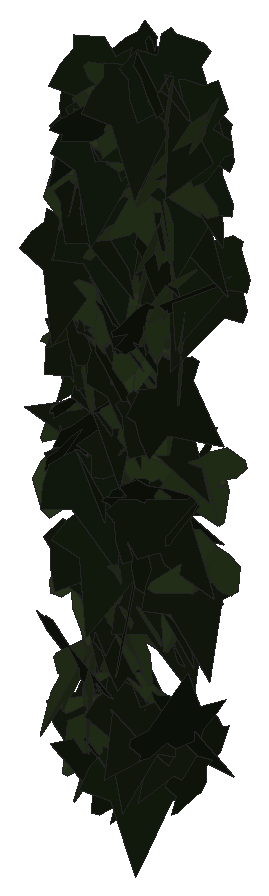
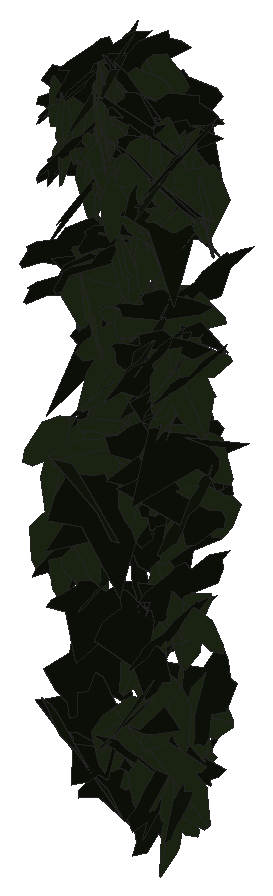
# SketchUp Ruby script. Lengths in inches.
U = 1.inch
M = Sketchup.active_model
def pt(a) = Geom::Point3d.new(a.map { |v| v * U })
def face(e, loops, mat)
  f = e.add_face(loops[0].map { |a| pt(a) })
  loops[1..].each { |l| e.add_face(l.map { |a| pt(a) }).erase! }
  f.material = f.back_material = mat if mat
  f
end
# faces: each face lists its corners as indices into pts; further lists are holes
def faces(e, pts, list, mat = nil) = list.each { |f| face(e, (f[0].is_a?(Array) ? f : [f]).map { |l| l.map { |i| pts[i] } }, mat) }
# xy, xz, yz: faces in a plane at the given z, y or x. An outline is a flat list of corners, or four numbers for a rectangle; further outlines are holes
def ring(l) = l.size == 4 ? [[l[0], l[1]], [l[2], l[1]], [l[2], l[3]], [l[0], l[3]]] : l.each_slice(2).to_a
def flat(e, list, mat, &to3) = list.each { |f| face(e, (f[0].is_a?(Array) ? f : [f]).map { |l| ring(l).map { |u, v| to3.(u, v) } }, mat) }
def xy(e, z, list, mat = nil) = flat(e, list, mat) { |x, y| [x, y, z] }
def xz(e, y, list, mat = nil) = flat(e, list, mat) { |x, z| [x, y, z] }
def yz(e, x, list, mat = nil) = flat(e, list, mat) { |y, z| [x, y, z] }
def lines(e, pts, list) = list.each { |a, b| e.add_line(pt(pts[a]), pt(pts[b])) }
# prism: a flat outline (further loops are holes) pulled along v
def prism(e, loops, v, mat = nil)
  f = face(e, loops, mat); d = Geom::Vector3d.new(v.map { |x| x * U })
  f.pushpull(f.normal.samedirection?(d) ? d.length : -d.length)
end
def box(e, o, s, mat = nil) = prism(e, [[o, [o[0] + s[0], o[1], o[2]], [o[0] + s[0], o[1] + s[1], o[2]], [o[0], o[1] + s[1], o[2]]]], [0, 0, s[2]], mat)
def at(x, y, z, deg = 0) = Geom::Transformation.translation(pt([x, y, z])) * Geom::Transformation.rotation(ORIGIN, Z_AXIS, deg.degrees)
def axes(o, x, y, z) = Geom::Transformation.new([*x, 0, *y, 0, *z, 0, *pt(o).to_a, 1])
def part(name) = M.definitions.add(name)
# library, detail: a bought-in or finely detailed component or shape, given as its bounding box
def library(name, o, s) = part(name).tap { |d| box(d.entities, o, s) }
def detail(e, o, s) = box(e.add_group.entities, o, s)
def put(e, d, t, mat = nil) = e.add_instance(d, t).tap { |i| i.material = mat if mat }
def group(e, t, mat = nil) = e.add_group.tap { |g| g.transformation = t; g.material = mat if mat }.entities
root = M.entities
M.materials.add("efeu1").color = [18, 25, 13]
M.materials.add("efeu2").color = [43, 57, 29]
c1 = part("ivyleaf_10")
p = [[0,0.5,-0.03],[-0.0625,2.02,-0.43],[-0.19,2.01,-0.46],[-0.54,1.05,-0.29],[-0.52,0.625,-0.18],[-0.83,0.76,-0.28],
  [-1.16,0.64,-0.33],[-1.15,0.33,-0.24],[-0.77,-0.39,0.02],[-0.3,-0.51,0.16],[0.04,-0.48,0.23],[-0.02,2.01,-0.4375],
  [-0.06,2.01,-0.43],[0.04,-0.49,0.23],[0.67,-0.49,0.14],[1.38,0.36,-0.2],[1.375,0.51,-0.24],[0.81,0.65,-0.19],
  [0.62,0.59,-0.15],[0.6,1.09,-0.28],[0.5,1.23,-0.31]]
faces(c1.entities,p,[[0,1,2,3,4,5,6,7,8,9,10],[11,12,0,13,14,15,16,17,18,19,20]],"efeu2")
c2 = part("ivyleaf_9")
p = [[1.54,2.16,1.25],[1.36,2.04,1.19],[-0.21,0.99,0.68],[-0.71,1.11,0.82],[-0.85,0.86,0.67],[-0.8,0.17,0.21],
  [-0.9,-0.01,0.1],[-0.67,-0.16,-0.02],[-0.08,-0.08,-0.05],[-0.03,-0.6,-0.4],[0.65,-0.88,-0.66],[0.83,-0.6,-0.49],
  [1.29,-0.42,-0.43],[1.8125,-0.07,-0.26],[1.21,0.44,0.15]]
faces(c2.entities,p,[[0,1,2,3,4,5,6,7,8,9,10,11,12,13,14]],"efeu1")
put(root,c1,axes([31.95,223.3,229.53],[-0.15216,-0.44786,0.16209],[-0.0246,-0.16254,-0.4722],[0.47565,-0.15167,0.02743]))
put(root,c1,axes([31.79,223.11,224.46],[0.10112,-0.23088,0.43182],[0.16851,-0.39759,-0.25203],[0.45976,0.19651,-0.0026]))
put(root,c1,axes([31.7,222.97,227.5],[0.1683,0.36123,0.30197],[0.14175,0.26693,-0.39832],[-0.44898,0.21968,-0.01256]))
put(root,c1,axes([31.99,223.31,223.23],[0.03537,-0.36052,-0.34463],[-0.03707,0.34264,-0.36225],[0.49737,0.05118,-0.00249]))
put(root,c2,axes([31.55,223.1875,224.62],[0.17291,-0.23827,0.40414],[0.26616,-0.30488,-0.29362],[0.38635,0.31667,0.0214]))
put(root,c2,axes([31.64,223.52,227.64],[0.15998,-0.38127,0.28113],[0.10465,-0.26095,-0.41346],[0.46201,0.19114,-0.00369]))
put(root,c2,axes([31.75,222.93,227.61],[0.21938,0.04053,0.44747],[0.27431,0.3823,-0.16911],[-0.35584,0.31969,0.1455]))
put(root,c1,axes([32.15,223.42,223.69],[-0.31593,-0.23667,0.30688],[-0.18778,-0.25286,-0.38833],[0.33901,-0.36062,0.07089]))
put(root,c2,axes([31.83,223.09,230.79],[-0.07401,-0.47877,0.12368],[-0.01118,-0.12341,-0.4844],[0.49437,-0.07447,0.00756]))
put(root,c2,axes([31.72,223.52,232.89],[0.20152,-0.45289,-0.06542],[-0.00268,0.07031,-0.49502],[0.45758,0.19987,0.02591]))
put(root,c1,axes([31.89,223.15,228.39],[-0.31509,-0.31993,-0.21992],[0.17985,0.13072,-0.44785],[0.34406,-0.36133,0.0327]))
put(root,c1,axes([32.01,222.82,232.1],[0.32533,-0.37423,-0.06411],[-0.0233,0.06459,-0.49526],[0.37897,0.32524,0.02459]))
put(root,c2,axes([31.97,223,228.66],[0.2119,0.40611,0.20043],[0.08645,0.18095,-0.45802],[-0.44455,0.22877,0.00647]))
put(root,c2,axes([31.79,223.6,231.4],[0.16857,-0.46772,0.05314],[0.02662,-0.04688,-0.49708],[0.46997,0.17042,0.0091]))
put(root,c1,axes([31.86,222.85,232],[-0.03215,-0.16781,-0.4699],[0.28412,0.38092,-0.15547],[0.41017,-0.27702,0.07086]))
put(root,c2,axes([31.85,223.22,229.45],[0.11041,-0.47255,-0.12046],[-0.02244,0.11845,-0.48525],[0.48714,0.11256,0.00495]))
put(root,c1,axes([31.88,223.23,225.96],[0.47699,-0.01024,0.14959],[0.14952,-0.00504,-0.47709],[0.01128,0.49987,-0.00175]))
put(root,c2,axes([31.91,223.15,226.53],[0.13506,-0.38024,-0.29526],[-0.04715,0.29473,-0.40113],[0.4791,0.13619,0.04375]))
put(root,c2,axes([32.23,223.125,223.68],[-0.4859,0.0659,0.09778],[0.09631,-0.01738,0.49033],[0.06803,0.49533,0.00419]))
put(root,c2,axes([31.95,223.57,225.81],[0.00346,-0.49008,0.09903],[0.00463,-0.09899,-0.49008],[0.49997,0.00431,0.00386]))
put(root,c2,axes([32.29,223.09,231.86],[-0.07124,0.49048,0.06597],[-0.00295,0.06622,-0.49559],[-0.49489,-0.071,-0.00654]))
put(root,c1,axes([32.09,223.15,229.08],[-0.14482,0.47251,0.07591],[-0.0215,0.07281,-0.4942],[-0.47808,-0.14641,-0.00077]))
put(root,c2,axes([31.97,222.81,228],[0.23281,0.15549,0.41427],[0.25312,0.33717,-0.2688],[-0.36295,0.33488,0.07828]))
put(root,c2,axes([32.3,223.51,230.46],[-0.4384,-0.22931,0.07224],[-0.0578,-0.0453,-0.49458],[0.23337,-0.442,0.01321]))
put(root,c1,axes([32.02,223.41,224.74],[-0.43035,0.13888,-0.21334],[0.19186,-0.09847,-0.4511],[-0.16731,-0.47012,0.03146]))
put(root,c2,axes([32.27,223.48,222.94],[-0.08389,0.04053,0.49124],[-0.28091,-0.4134,-0.01386],[0.40504,-0.27831,0.09213]))
put(root,c2,axes([32.54,223.41,228.09],[-0.21093,0.02475,0.45266],[-0.44867,-0.08283,-0.20454],[0.06486,-0.49247,0.05715]))
put(root,c2,axes([32.05,223.57,222.91],[0.37703,-0.31657,-0.08736],[0.08514,-0.03424,0.49151],[-0.31718,-0.3855,0.02809]))
put(root,c1,axes([32.37,223.28,230.375],[-0.45321,-0.14291,0.15548],[-0.15242,-0.03344,-0.47503],[0.14617,-0.47797,-0.01325]))
put(root,c2,axes([31.96,223.1875,229.7],[0.29462,-0.38629,-0.11824],[-0.03557,0.12097,-0.48384],[0.40241,0.29351,0.0438]))
put(root,c2,axes([31.97,223.5,232.58],[0.31969,-0.37256,-0.09486],[-0.04991,0.08211,-0.49068],[0.38119,0.3232,0.01531]))
put(root,c2,axes([32.06,223.06,227.66],[-0.00638,-0.44383,-0.23017],[0.00872,0.23006,-0.44384],[0.49988,-0.00968,0.0048]))
put(root,c1,axes([32.34,222.97,230.21],[-0.43727,-0.21936,0.10331],[-0.07112,-0.08764,-0.48709],[0.23181,-0.44068,0.04545]))
put(root,c2,axes([32.15,223.5,233.49],[-0.28871,-0.35947,-0.19347],[0.1448,0.13138,-0.46019],[0.38168,-0.32175,0.02824]))
put(root,c1,axes([32.3,223.3125,232.61],[-0.26649,-0.42009,-0.05009],[0.02341,0.04447,-0.49747],[0.42242,-0.26748,-0.00404]))
put(root,c2,axes([32.39,223.47,229.81],[-0.42595,-0.25919,0.03727],[-0.03158,-0.01979,-0.49861],[0.25995,-0.42712,0.00049]))
put(root,c2,axes([32.65,223.3,232.27],[-0.2754,0.27364,0.31508],[-0.27936,0.15956,-0.38275],[-0.31002,-0.38686,0.06501]))
put(root,c1,axes([32.1,223.05,224.53],[0.26512,-0.32868,0.26773],[0.23185,-0.15195,-0.41612],[0.3549,0.3448,0.07184]))
put(root,c2,axes([32.48,223.24,232.01],[-0.49476,-0.04568,-0.05589],[0.05795,-0.0205,-0.49621],[0.04305,-0.49749,0.02558]))
put(root,c2,axes([32.5,222.86,233.12],[-0.04445,0.34381,-0.36031],[-0.0127,-0.3624,-0.34424],[-0.49786,-0.02145,0.04095]))
put(root,c2,axes([32.17,223.66,229.76],[0.04,-0.49839,-0.00276],[-0.00296,0.00253,-0.49998],[0.49839,0.04001,-0.00275]))
put(root,c2,axes([32.14,223.39,228.64],[0.11426,-0.46594,0.14088],[0.0383,-0.13566,-0.47972],[0.48526,0.12042,0.0047]))
put(root,c1,axes([32.25,223.07,225.62],[-0.44278,-0.02898,0.23046],[0.23198,-0.03036,0.44189],[-0.01162,0.49824,0.04033]))
put(root,c2,axes([32.24,223.33,225.1],[0.34239,-0.24469,-0.26999],[-0.17881,0.20997,-0.41706],[0.31748,0.38215,0.05627]))
put(root,c2,axes([32.39,223.31,232.8],[-0.29893,-0.39819,-0.04565],[0.02172,0.04078,-0.49786],[0.40021,-0.29963,-0.00708]))
put(root,c2,axes([32.2,222.85,231.76],[0.24039,-0.41808,-0.13199],[-0.03507,0.13171,-0.48106],[0.43701,0.24055,0.034]))
put(root,c1,axes([32.59,223.27,233.03],[-0.47213,0.02859,0.16209],[-0.16181,0.0094,-0.473],[-0.03009,-0.49909,0.00038]))
put(root,c1,axes([32.6875,223.5,224.16],[-0.31464,-0.20558,0.32976],[-0.26089,-0.20271,-0.3753],[0.28799,-0.40823,0.02029]))
put(root,c1,axes([32.64,222.87,233.43],[0.33344,-0.14115,-0.34481],[-0.26808,0.23047,-0.35358],[0.25875,0.42067,0.07801]))
put(root,c1,axes([32.26,223.03,233.09],[-0.38063,0.02859,-0.32296],[0.31849,-0.06025,-0.3807],[-0.06069,-0.49553,0.02765]))
put(root,c2,axes([32.37,223.0625,232.56],[-0.06549,-0.49256,0.05561],[-0.00587,-0.05532,-0.4969],[0.49566,-0.06574,0.00147]))
put(root,c1,axes([32.52,223.75,232.21],[-0.03355,-0.43938,0.23627],[0.0328,-0.23823,-0.43837],[0.49779,-0.01391,0.04481]))
put(root,c1,axes([32.4,223.69,227.51],[0.03696,-0.26143,-0.42461],[0.04732,-0.42201,0.26395],[-0.49638,-0.0597,-0.00646]))
put(root,c1,axes([32.38,222.9,223.96],[-0.35955,-0.21336,-0.27423],[0.24469,0.12468,-0.41783],[0.24668,-0.43466,0.01476]))
put(root,c1,axes([32.51,223.16,231.16],[0.05607,-0.46461,0.17604],[0.07207,-0.16768,-0.4655],[0.49159,0.07758,0.04817]))
put(root,c2,axes([32.35,223.23,230.04],[0.36254,-0.30862,-0.15271],[-0.11979,0.09485,-0.47608],[0.32283,0.38178,-0.00516]))
put(root,c2,axes([32.84,223.54,233.15],[-0.48843,0.07124,0.07975],[-0.08617,-0.04138,-0.49078],[-0.06333,-0.49317,0.0527]))
put(root,c2,axes([32.54,223.14,226.78],[-0.28293,-0.40885,-0.05284],[0.02137,0.04945,-0.49709],[0.4117,-0.28354,-0.01051]))
put(root,c1,axes([32.86,223.11,233.15],[0.22696,-0.00918,-0.44543],[-0.41459,0.17867,-0.21493],[0.16311,0.4669,0.07349]))
put(root,c2,axes([32.43,222.9375,231.47],[-0.02031,-0.46828,-0.17408],[0.00454,0.17404,-0.46871],[0.49957,-0.02062,-0.00282]))
put(root,c1,axes([32.55,223.23,225.48],[-0.46074,0.16534,-0.10191],[0.09308,-0.04228,-0.48944],[-0.17047,-0.46997,0.00818]))
put(root,c2,axes([32.74,223.49,233.68],[-0.47354,0.0706,-0.14414],[0.14494,-0.00476,-0.47851],[-0.06894,-0.49497,-0.01596]))
put(root,c2,axes([32.375,223.3,229.12],[0.16211,-0.46712,0.0743],[0.02677,-0.06935,-0.49444],[0.47223,0.16428,0.00253]))
put(root,c2,axes([32.24,223.57,225.61],[0.06773,-0.07357,-0.4899],[0.47317,0.15605,0.04198],[0.14672,-0.46929,0.09076]))
put(root,c1,axes([32.65,223.29,231.77],[-0.19415,-0.45201,-0.08938],[0.07166,0.06619,-0.49039],[0.45516,-0.20323,0.03908]))
put(root,c2,axes([32.6,223.74,231.66],[-0.21276,-0.45199,0.02106],[-0.00654,-0.0202,-0.49955],[0.45243,-0.21284,0.00269]))
put(root,c2,axes([32.37,223.16,230.21],[0.36883,-0.3353,0.03921],[0.03263,-0.0224,-0.49843],[0.336,0.37024,0.00535]))
put(root,c1,axes([32.89,223.48,232.27],[0.07656,0.16839,0.46453],[-0.22434,-0.40698,0.1845],[0.44024,-0.23667,0.01324]))
put(root,c2,axes([32.47,222.98,229.35],[0.41716,-0.26747,-0.06659],[-0.06583,0.02063,-0.49522],[0.26766,0.42194,-0.018]))
put(root,c1,axes([32.73,223.28,229.91],[0.49349,0.07774,0.02058],[0.02035,0.00309,-0.49958],[-0.0778,0.49391,-0.00011]))
put(root,c1,axes([32.96,223.14,228.6],[-0.43297,-0.22707,0.10476],[-0.08365,-0.06588,-0.48853],[0.23566,-0.44057,0.01906]))
put(root,c2,axes([32.78,223.4,224.06],[-0.13098,-0.37834,0.29951],[-0.00632,-0.30897,-0.39306],[0.4825,-0.10675,0.07616]))
put(root,c1,axes([32.7,223.35,232.2],[0.40878,-0.17947,0.22515],[0.20861,-0.08488,-0.4464],[0.19845,0.4589,0.00548]))
put(root,c2,axes([32.82,223.27,223.33],[-0.19345,-0.43912,-0.14054],[0.04573,0.13339,-0.4797],[0.45879,-0.19845,-0.01145]))
put(root,c2,axes([33.03,223.58,223.77],[-0.47545,-0.12824,-0.08659],[0.08613,0.0131,-0.49235],[0.12855,-0.4831,0.00964]))
put(root,c2,axes([32.8,223.19,224.14],[-0.04658,-0.48657,0.10526],[0.00142,-0.10585,-0.48867],[0.49782,-0.04523,0.01124]))
put(root,c1,axes([33.16,223.65,230.66],[0.09181,0.19992,-0.449],[-0.36784,-0.275,-0.19766],[-0.32599,0.36661,0.09658]))
put(root,c2,axes([32.85,223.08,226.375],[-0.23196,0.10952,-0.42919],[0.39825,-0.16049,-0.2562],[-0.19388,-0.4607,-0.01278]))
put(root,c2,axes([33.1,223.31,227.49],[0.21803,0.36441,-0.26395],[-0.19466,-0.18805,-0.42041],[-0.40568,0.28608,0.05987]))
put(root,c1,axes([33,223.4,232.53],[0.47729,-0.08557,-0.12197],[-0.10362,0.10346,-0.47808],[0.10706,0.48164,0.08103]))
put(root,c1,axes([32.87,223.25,229.57],[-0.26397,-0.32314,-0.2755],[0.22435,0.16929,-0.41353],[0.36054,-0.34193,0.05562]))
put(root,c1,axes([32.98,223.43,231.2],[0.4254,-0.25382,-0.06787],[-0.04284,0.06043,-0.49448],[0.25922,0.42652,0.02967]))
put(root,c1,axes([32.78,223.01,232.83],[-0.29469,-0.15233,-0.3741],[0.34613,0.14346,-0.33108],[0.2082,-0.45411,0.02091]))
put(root,c1,axes([33.04,223.47,233.48],[0.17343,-0.45776,-0.10189],[-0.00046,0.10847,-0.48809],[0.46896,0.16939,0.0372]))
put(root,c2,axes([32.83,223.01,227.4],[0.45515,0.15152,0.14099],[0.13225,0.04909,-0.47969],[-0.1592,0.47395,0.00461]))
put(root,c2,axes([32.91,223.32,233.8],[0.36181,-0.28703,-0.1916],[-0.13976,0.13194,-0.46158],[0.31553,0.38757,0.01524]))
put(root,c2,axes([33.05,223.67,230.9],[-0.18022,-0.4645,0.04197],[0.00717,-0.04775,-0.49766],[0.46633,-0.17878,0.02388]))
put(root,c1,axes([33.15,223.43,233.13],[0.21504,-0.45021,-0.03276],[0.03151,0.05117,-0.49637],[0.4503,0.21141,0.05038]))
put(root,c2,axes([33.0625,222.95,233.63],[-0.1311,-0.47507,-0.08438],[0.01517,0.08334,-0.49277],[0.48227,-0.13176,-0.00744]))
put(root,c2,axes([33.04,223.45,225.95],[-0.13382,-0.37427,-0.30333],[0.11583,0.28059,-0.39731],[0.46763,-0.17661,0.01161]))
put(root,c1,axes([33.27,223.46,230.46],[0.16127,-0.46664,-0.07901],[-0.02509,0.07492,-0.49372],[0.47261,0.16321,0.00075]))
put(root,c2,axes([33.06,223.32,233.92],[0.16026,-0.34906,-0.32012],[-0.00917,0.3356,-0.37053],[0.47353,0.12463,0.10116]))
put(root,c2,axes([33.16,223.04,231.43],[0.32463,-0.26467,-0.27307],[-0.19729,0.18972,-0.41843],[0.3251,0.37942,0.01874]))
put(root,c1,axes([33.28,222.94,231.54],[0.236,-0.4373,0.0554],[0.02973,-0.04691,-0.49691],[0.4398,0.23783,0.00386]))
put(root,c2,axes([33.3,223.16,227.07],[-0.29992,0.39998,-0.00817],[-0.00645,0.00538,0.49993],[0.40001,0.29998,0.00194]))
put(root,c2,axes([33.02,223.28,226.33],[0.24236,-0.42968,0.08147],[0.04945,-0.06562,-0.4932],[0.43453,0.24713,0.01069]))
put(root,c1,axes([32.98,223.22,228.02],[-0.14053,-0.10865,-0.46738],[0.46117,0.10398,-0.16283],[0.13258,-0.47685,0.07099]))
put(root,c2,axes([33.11,222.69,230.14],[0.08969,0.45139,-0.19547],[0.03782,0.19177,0.46021],[0.49043,-0.09734,0.00025]))
put(root,c1,axes([33.41,222.93,228.61],[-0.06152,0.43497,-0.23879],[-0.02823,0.23716,0.43927],[0.4954,0.06753,-0.00462]))
put(root,c1,axes([33.3125,222.82,232.11],[-0.12693,-0.47503,-0.09076],[0.10973,0.06309,-0.48371],[0.47101,-0.14271,0.08823]))
put(root,c1,axes([33.21,223.28,233.4],[0.30992,-0.35414,0.16891],[0.17371,-0.06916,-0.46373],[0.35181,0.34612,0.08017]))
put(root,c1,axes([33.38,223.09,230.55],[0.0732,-0.47375,-0.14215],[0.01446,0.14569,-0.47809],[0.4944,0.06588,0.03503]))
put(root,c2,axes([33.12,223.11,228.85],[0.19585,-0.41943,-0.18901],[0.01317,0.21045,-0.45336],[0.45986,0.1726,0.09348]))
put(root,c1,axes([33.51,222.86,231.95],[-0.33171,0.35397,0.12113],[-0.20455,-0.03606,-0.45482],[-0.31325,-0.35129,0.16873]))
put(root,c2,axes([33.08,223.03,227.36],[-0.082,-0.13887,-0.47328],[0.3419,0.3298,-0.15601],[0.3555,-0.34921,0.04087]))
put(root,c1,axes([33.42,223.01,232.68],[0.01932,-0.46,-0.19501],[0.00884,0.19544,-0.46014],[0.49955,0.01433,0.01569]))
put(root,c1,axes([33.45,222.86,230.48],[0.05043,0.30544,0.39264],[-0.16157,0.38331,-0.27743],[-0.47048,-0.09889,0.13736]))
put(root,c2,axes([33.03,223.51,223.97],[0.22181,0.04837,-0.44549],[0.43885,0.07708,0.22687],[0.09062,-0.49165,-0.00826]))
put(root,c1,axes([33.52,222.99,232.24],[-0.46806,-0.17538,0.01256],[-0.01172,-0.00451,-0.49984],[0.17544,-0.46821,0.00011]))
put(root,c2,axes([33.77,223.43,233.08],[-0.36682,-0.13824,0.31037],[-0.2934,-0.10145,-0.39195],[0.17134,-0.46968,-0.00669]))
put(root,c2,axes([33.28,223.38,231.89],[0.26135,-0.38237,-0.18837],[-0.07958,0.17331,-0.4622],[0.41876,0.27158,0.02973]))
put(root,c2,axes([33.8125,223.27,223.64],[-0.30772,0.34814,0.18469],[-0.12813,0.1332,-0.46458],[-0.37268,-0.33325,0.00724]))
put(root,c1,axes([33.76,223.46,226.68],[-0.38213,-0.1254,0.29707],[-0.26693,-0.13541,-0.40052],[0.1809,-0.46469,0.03654]))
put(root,c2,axes([33.3,223.625,232.66],[0.14556,-0.4696,-0.09102],[-0.001,0.09484,-0.49092],[0.47834,0.1431,0.02667]))
put(root,c2,axes([33.47,223.83,230.64],[-0.19558,-0.45049,0.09387],[0.00419,-0.10374,-0.4891],[0.46014,-0.19053,0.04436]))
put(root,c2,axes([33.54,223.75,231.11],[-0.21457,-0.4508,0.02716],[0.00855,-0.03412,-0.49876],[0.45154,-0.21357,0.02235]))
put(root,c1,axes([33.46,223.27,230.1],[0.29991,-0.33692,0.21573],[0.19445,-0.11287,-0.4466],[0.34964,0.35177,0.06333]))
put(root,c2,axes([33.52,223.43,232.33],[-0.09294,-0.48971,0.03935],[-0.00424,-0.03924,-0.49844],[0.49127,-0.09299,0.00314]))
put(root,c2,axes([33.55,222.68,229.43],[0.13824,-0.17762,-0.44648],[-0.18963,0.40671,-0.22051],[0.44151,0.2303,0.04509]))
put(root,c1,axes([33.67,223.3,226.36],[-0.10186,-0.4244,0.24395],[0.02466,-0.25331,-0.43038],[0.48889,-0.07564,0.07254]))
put(root,c1,axes([33.66,223.4375,232.91],[0.12484,-0.45168,-0.17435],[0.02769,0.18642,-0.46312],[0.48337,0.10597,0.07156]))
put(root,c1,axes([33.71,223.38,233.15],[0.02896,-0.49575,-0.05829],[-0.01095,0.05774,-0.49653],[0.49904,0.03003,-0.00751]))
put(root,c2,axes([33.59,223.5625,233.125],[-0.12952,-0.41868,0.24068],[0.00449,-0.25022,-0.43286],[0.48291,-0.10997,0.06857]))
put(root,c1,axes([33.71,223.39,227.99],[-0.28007,-0.39559,-0.12275],[0.08393,0.0909,-0.48445],[0.4056,-0.29197,0.01548]))
put(root,c2,axes([33.56,223.29,226.47],[0.0227,-0.47384,-0.15799],[-0.01375,0.1575,-0.47434],[0.4993,0.02588,-0.00588]))
put(root,c2,axes([33.57,222.84,224.14],[0.27101,0.33477,0.25394],[-0.15713,-0.19951,0.4307],[0.3897,-0.31325,-0.00293]))
